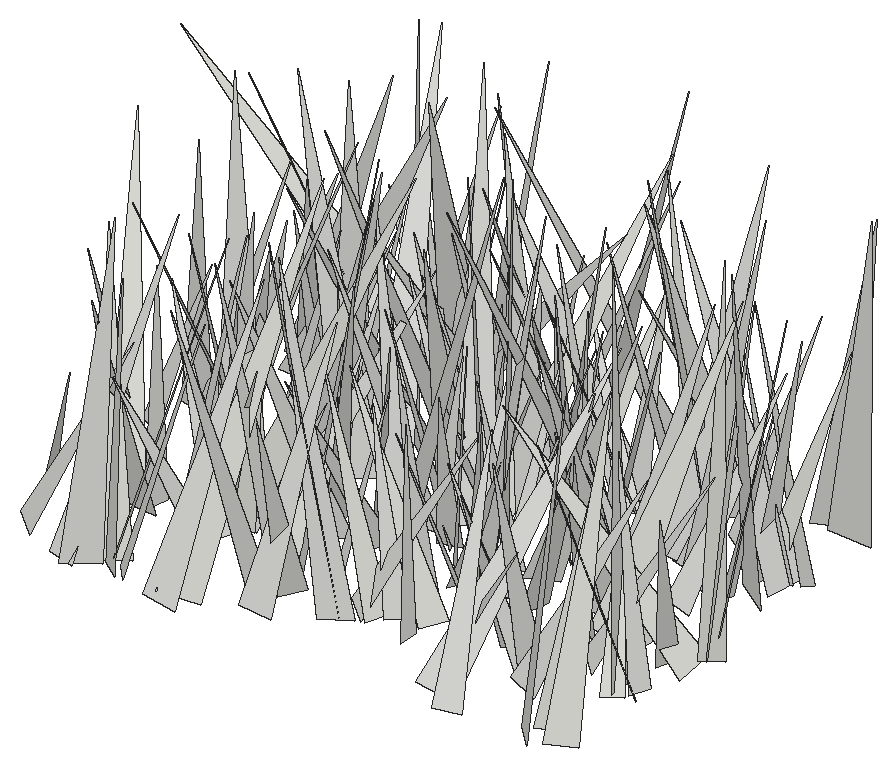
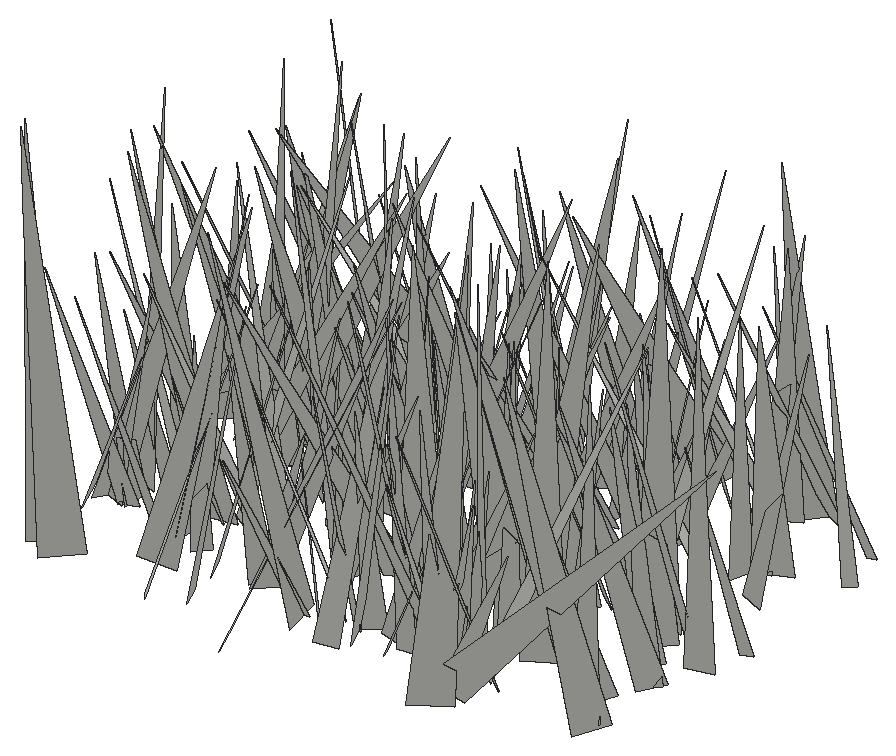
# SketchUp Ruby script. Lengths in inches.
U = 1.inch
M = Sketchup.active_model
def pt(a) = Geom::Point3d.new(a.map { |v| v * U })
def face(e, loops, mat)
  f = e.add_face(loops[0].map { |a| pt(a) })
  loops[1..].each { |l| e.add_face(l.map { |a| pt(a) }).erase! }
  f.material = f.back_material = mat if mat
  f
end
# faces: each face lists its corners as indices into pts; further lists are holes
def faces(e, pts, list, mat = nil) = list.each { |f| face(e, (f[0].is_a?(Array) ? f : [f]).map { |l| l.map { |i| pts[i] } }, mat) }
# xy, xz, yz: faces in a plane at the given z, y or x. An outline is a flat list of corners, or four numbers for a rectangle; further outlines are holes
def ring(l) = l.size == 4 ? [[l[0], l[1]], [l[2], l[1]], [l[2], l[3]], [l[0], l[3]]] : l.each_slice(2).to_a
def flat(e, list, mat, &to3) = list.each { |f| face(e, (f[0].is_a?(Array) ? f : [f]).map { |l| ring(l).map { |u, v| to3.(u, v) } }, mat) }
def xy(e, z, list, mat = nil) = flat(e, list, mat) { |x, y| [x, y, z] }
def xz(e, y, list, mat = nil) = flat(e, list, mat) { |x, z| [x, y, z] }
def yz(e, x, list, mat = nil) = flat(e, list, mat) { |y, z| [x, y, z] }
def lines(e, pts, list) = list.each { |a, b| e.add_line(pt(pts[a]), pt(pts[b])) }
# prism: a flat outline (further loops are holes) pulled along v
def prism(e, loops, v, mat = nil)
  f = face(e, loops, mat); d = Geom::Vector3d.new(v.map { |x| x * U })
  f.pushpull(f.normal.samedirection?(d) ? d.length : -d.length)
end
def box(e, o, s, mat = nil) = prism(e, [[o, [o[0] + s[0], o[1], o[2]], [o[0] + s[0], o[1] + s[1], o[2]], [o[0], o[1] + s[1], o[2]]]], [0, 0, s[2]], mat)
def at(x, y, z, deg = 0) = Geom::Transformation.translation(pt([x, y, z])) * Geom::Transformation.rotation(ORIGIN, Z_AXIS, deg.degrees)
def axes(o, x, y, z) = Geom::Transformation.new([*x, 0, *y, 0, *z, 0, *pt(o).to_a, 1])
def part(name) = M.definitions.add(name)
# library, detail: a bought-in or finely detailed component or shape, given as its bounding box
def library(name, o, s) = part(name).tap { |d| box(d.entities, o, s) }
def detail(e, o, s) = box(e.add_group.entities, o, s)
def put(e, d, t, mat = nil) = e.add_instance(d, t).tap { |i| i.material = mat if mat }
def group(e, t, mat = nil) = e.add_group.tap { |g| g.transformation = t; g.material = mat if mat }.entities
root = M.entities
c1 = part("fur_instance\#9")
p = [[0.8125,0,1.79],[0.67,-0.02,1.48],[0,-0.11,0],[0,0.11,0]]
faces(c1.entities,p,[[0,1,2,3]])
put(root,c1,axes([91.07,234.39,-27.1],[4.75602,-4.66812,2.75377],[-5.20371,-4.95731,0.58378],[-1.51526,2.37234,6.63855]))
put(root,c1,axes([111.02,234.4375,-27.1],[4.54729,4.68314,2.12923],[4.88324,-4.82336,0.17985],[-1.61844,-1.39522,6.52513]))
put(root,c1,axes([92.14,234.72,-27.1],[3.06348,4.37723,2.06786],[4.6001,-3.39453,0.37061],[-1.50841,-1.46222,5.32989]))
put(root,c1,axes([97.12,236.8125,-27.1],[-5.96376,-1.66281,1.60864],[-1.32131,6.09893,1.40577],[1.89916,-0.97833,6.02952]))
put(root,c1,axes([98.24,237.36,-27.1],[3.42227,-3.49613,0.30492],[-3.40506,-3.41104,-0.89344],[-0.84941,-0.41195,4.81005]))
put(root,c1,axes([94.98,233.9,-27.1],[0.10942,6.44965,1.02032],[6.44115,0.06102,-1.07648],[1.07264,-1.02435,6.36012]))
put(root,c1,axes([87.73,235.44,-27.1],[2.82226,4.09729,0.68802],[3.94816,-2.38599,-1.98631],[1.29353,-1.65697,4.56152]))
put(root,c1,axes([107.76,234.14,-27.1],[-1.60174,4.9541,0.61833],[4.97114,1.64265,-0.28364],[0.46172,-0.4996,5.19887]))
put(root,c1,axes([87.05,237.49,-27.1],[4.69242,0.16576,0.10905],[0.19618,-4.2622,-1.96297],[-0.02968,-1.96577,4.26532]))
put(root,c1,axes([92.63,234.77,-27.1],[3.7464,3.46532,0.67043],[3.46985,-3.79505,0.22613],[-0.64655,-0.28736,5.09832]))
put(root,c1,axes([91.81,235.25,-27.1],[-3.36286,5.21282,1.50099],[5.38655,3.41774,0.19865],[0.64152,-1.37145,6.20023]))
put(root,c1,axes([105.42,237.17,-27.1],[3.7363,2.07589,0.22504],[1.88074,-3.14536,-2.2112],[0.90706,-2.02911,3.65784]))
put(root,c1,axes([90.27,238.74,-27.1],[0.60186,-6.09784,0.10298],[-6.0697,-0.58883,0.60707],[0.59415,0.16161,6.09732]))
put(root,c1,axes([93.92,237.96,-27.1],[-4.12735,0.23871,1.0618],[0.66209,3.85593,1.70672],[0.86374,-1.81501,3.76552]))
put(root,c1,axes([98.04,235.48,-27.1],[-0.68675,5.73435,1.62653],[5.78722,1.03346,-1.2],[1.42703,-1.4315,5.64928]))
put(root,c1,axes([108.55,237.99,-27.1],[4.51587,-1.82573,1.61231],[-1.49442,-4.75873,-1.20297],[-1.92343,-0.58918,4.72009]))
put(root,c1,axes([90.3125,234.2,-27.1],[2.22729,6.28936,0.04999],[6.2767,-2.22605,0.40869],[-0.40191,0.08939,6.65956]))
put(root,c1,axes([100.12,237.37,-27.1],[4.02018,4.80904,4.066],[5.52928,-5.00439,0.45193],[-3.01434,-2.76593,6.25176]))
put(root,c1,axes([94.29,235.29,-27.1],[4.06792,5.19434,1.22411],[5.14399,-4.22635,0.83955],[-1.42088,-0.42943,6.54403]))
put(root,c1,axes([100.61,236.82,-27.1],[0.55965,-6.1533,3.26603],[-6.71098,-1.35523,-1.40332],[-1.86889,3.02383,6.01722]))
put(root,c1,axes([112.45,234.71,-27.1],[-5.42402,3.35952,0.54018],[3.08821,5.28712,-1.87283],[1.42868,1.32596,6.09909]))
put(root,c1,axes([106.79,239.1,-27.1],[1.2889,-4.23263,0.01136],[-4.22076,-1.28617,-0.32791],[-0.31699,-0.08469,4.41236]))
put(root,c1,axes([111.32,235.29,-27.1],[-4.3486,2.21974,0.80785],[1.83051,4.23636,-1.78683],[1.49303,1.27131,4.54366]))
put(root,c1,axes([103.45,237.36,-27.1],[-3.94466,-0.14605,1.57067],[-0.23954,4.23653,-0.20765],[1.55915,0.28136,3.94189]))
put(root,c1,axes([111.99,239.29,-27.1],[-3.65311,-4.50937,0.62916],[-4.48426,3.70309,0.50402],[0.78847,0.16789,5.78149]))
put(root,c1,axes([108.77,237.1,-27.1],[0.87918,5.14411,1.43079],[4.85097,-0.16366,-2.39235],[2.23095,-1.67133,4.63805]))
put(root,c1,axes([108.61,237.67,-27.1],[-0.27177,-3.75184,1.87256],[-3.70908,-0.66019,-1.86105],[-1.95589,1.77327,3.26904]))
put(root,c1,axes([96.52,238.8,-27.1],[-6.02473,-0.71032,1.74625],[-0.51818,6.24626,0.75302],[1.81257,-0.57532,6.01954]))
put(root,c1,axes([101.71,237.83,-27.1],[-4.44101,1.77663,0.66677],[1.83519,4.45274,0.3588],[0.48276,-0.58331,4.76973]))
put(root,c1,axes([106.6,234.94,-27.1],[-2.65177,6.66161,0.65253],[5.97681,2.67255,-2.995],[3.01341,0.56142,6.51452]))
put(root,c1,axes([100.72,237.83,-27.1],[2.95433,4.07724,0.35212],[3.82019,-2.59183,-2.04072],[1.46767,-1.46099,4.60298]))
put(root,c1,axes([93.55,238.49,-27.1],[4.21997,-0.6182,0.41958],[-0.60999,-4.24047,-0.11271],[-0.43142,-0.05127,4.26352]))
put(root,c1,axes([104.69,239.23,-27.1],[5.27182,0.13194,1.25121],[0.40362,-5.28245,-1.14356],[-1.19165,-1.2055,5.14798]))
put(root,c1,axes([95.3,234.58,-27.1],[-5.76444,5.45156,1.05869],[4.71185,5.60881,-3.22628],[2.93919,1.70025,7.24841]))
put(root,c1,axes([102.25,238.19,-27.1],[-2.34318,3.21724,1.23905],[3.43189,2.31946,0.46753],[0.3286,-1.2829,3.95253]))
put(root,c1,axes([91.68,235.6,-27.1],[4.88269,3.53574,0.69101],[3.04894,-4.67553,2.3797],[-1.91908,1.56767,5.53887]))
put(root,c1,axes([103.54,238.68,-27.1],[-3.16425,3.77948,0.90882],[3.82647,2.82214,1.58634],[-0.68447,-1.69527,4.66695]))
put(root,c1,axes([90.54,239.28,-27.1],[4.66089,-0.94094,1.87831],[-0.93791,-5.02216,-0.1885],[-1.87983,0.17273,4.75118]))
put(root,c1,axes([99.8,237.57,-27.1],[2.15657,3.40289,0.33157],[3.29952,-2.17412,0.8525],[-0.89598,0.18416,3.93747]))
put(root,c1,axes([93.79,238.93,-27.1],[-4.37438,2.14658,0.79892],[2.22863,4.38643,0.41683],[0.52851,-0.72986,4.85482]))
put(root,c1,axes([106.63,236.22,-27.1],[4.76717,4.34009,0.09976],[4.0907,-4.54047,2.05487],[-1.45344,1.45601,6.11063]))
put(root,c1,axes([104.82,239.42,-27.1],[-3.19994,-2.12817,0.10035],[-2.08753,3.09569,-0.91527],[-0.42587,0.81635,3.73243]))
put(root,c1,axes([94.13,239.69,-27.1],[2.50338,-2.82714,1.30611],[-3.05988,-2.54469,0.35667],[-0.57944,1.22368,3.75931]))
put(root,c1,axes([89.07,240.52,-27.1],[-1.67954,-4.60165,1.09216],[-4.72861,1.65608,-0.29411],[0.09072,1.12742,4.88974]))
put(root,c1,axes([93.97,240.62,-27.1],[-1.02707,-3.52995,0.46815],[-3.49734,0.90838,-0.82343],[-0.66956,0.66999,3.58293]))
put(root,c1,axes([101.92,240.24,-27.1],[0.28904,-4.61969,1.68996],[-4.89331,-0.44312,-0.3744],[-0.50298,1.65624,4.61355]))
put(root,c1,axes([111.68,238.54,-27.1],[-2.57238,2.98987,0.10946],[2.97729,2.57237,-0.29516],[0.29502,0.10983,3.93311]))
put(root,c1,axes([98.65,241.95,-27.1],[1.56687,-4.2825,0.24372],[-4.04586,-1.5617,-1.43053],[-1.42486,-0.27491,4.32996]))
put(root,c1,axes([112.21,239.42,-27.1],[-4.36363,0.98227,0.81119],[0.91976,4.432,-0.41906],[0.88144,0.23814,4.45315]))
put(root,c1,axes([97.375,238.89,-27.1],[5.30824,4.83924,1.79848],[4.88732,-5.54151,0.48577],[-1.6634,-0.83881,7.16657]))
put(root,c1,axes([97.09,241.42,-27.1],[0.61294,-5.47928,1.38132],[-5.30961,-1.0339,-1.7451],[-1.93355,1.10218,5.22999]))
put(root,c1,axes([111.69,241.67,-27.1],[3.7269,-2.05729,0.24824],[-1.97365,-3.67974,-0.86491],[-0.63149,-0.64103,4.16823]))
put(root,c1,axes([112.61,241.98,-27.1],[-5.96221,1.49508,0.02596],[1.36332,5.39133,2.61894],[-0.61423,-2.54602,5.56097]))
put(root,c1,axes([109.48,239.97,-27.1],[3.29682,4.04593,0.27696],[3.82738,-2.98619,-1.93627],[1.34069,-1.42422,4.84659]))
put(root,c1,axes([111.5,239.28,-27.1],[-7.33304,-1.55705,2.53328],[-2.07568,7.50758,-1.39398],[2.1292,1.95633,7.36578]))
put(root,c1,axes([107.93,241.74,-27.1],[-3.27673,-6.38483,2.25273],[-6.55108,3.62196,0.73666],[1.71005,1.64109,7.13865]))
put(root,c1,axes([96.43,242.04,-27.1],[6.1777,-0.38175,1.16241],[-0.13775,-6.16226,-1.29169],[-1.21571,-1.24165,6.0532]))
put(root,c1,axes([108.61,243.0625,-27.1],[1.25653,-6.81976,0.6894],[-6.81087,-1.32116,-0.65555],[-0.77223,0.55558,6.90349]))
put(root,c1,axes([89.71,238.5,-27.1],[-3.35316,6.39569,0.22234],[6.39729,3.34326,0.30873],[-0.17041,-0.34016,7.2148]))
put(root,c1,axes([92.72,241.87,-27.1],[-4.52954,-3.25843,1.35312],[-3.24257,4.71245,0.49358],[1.39071,0.3748,5.55792]))
put(root,c1,axes([90.9,244.39,-27.1],[-3.5223,-6.70382,0.02091],[-6.50166,3.42181,1.83516],[1.63401,-0.83562,7.34711]))
put(root,c1,axes([105.59,241.77,-27.1],[5.75538,-1.33671,0.29214],[-1.31847,-5.75568,-0.36093],[-0.36579,-0.28603,5.89753]))
put(root,c1,axes([96.39,239.39,-27.1],[-0.08905,4.06249,0.07241],[4.03019,0.09752,-0.5148],[0.51634,-0.06053,4.03072]))
put(root,c1,axes([96.22,240.78,-27.1],[6.38411,4.40631,2.11358],[4.61615,-6.57865,-0.22824],[-1.60436,-1.39477,7.75373]))
put(root,c1,axes([97.61,242.99,-27.1],[4.97524,0.71585,1.07536],[1.04452,-4.74693,-1.67259],[-0.76015,-1.83742,4.74004]))
put(root,c1,axes([110.31,242.54,-27.1],[-3.89042,0.9571,1.21715],[1.27935,3.84105,1.06884],[0.87221,-1.36496,3.86121]))
put(root,c1,axes([93.42,240.59,-27.1],[2.59444,7.48207,1.23534],[7.31718,-2.12705,-2.48457],[1.99156,-1.93206,7.51927]))
put(root,c1,axes([100.42,243.47,-27.1],[1.67975,-3.93598,0.16611],[-3.93538,-1.66827,0.26597],[0.17974,0.25696,4.27115]))
put(root,c1,axes([100.32,241.13,-27.1],[-1.21025,6.4146,1.42422],[6.45546,0.89059,1.47445],[-1.22575,-1.64315,6.35907]))
put(root,c1,axes([91.96,239.77,-27.1],[5.80303,5.01805,0.27093],[4.96083,-5.78629,0.91567],[-0.80277,0.51711,7.61693]))
put(root,c1,axes([107.73,242.9,-27.1],[0.85171,-3.4207,0.8533],[-3.50883,-0.73716,0.54719],[0.34265,0.95401,3.48241]))
put(root,c1,axes([101.58,242.3125,-27.1],[3.14318,2.78213,1.66083],[2.96777,-3.40061,0.07991],[-1.30037,-1.03624,4.19683]))
put(root,c1,axes([103.09,241.92,-27.1],[4.37398,5.97616,2.1686],[6.29129,-4.44766,-0.43255],[-0.91492,-2.01317,7.39318]))
put(root,c1,axes([102.34,241.34,-27.1],[4.56042,0.58445,0.815],[0.35248,-4.48653,1.24501],[-0.93891,1.15443,4.42595]))
put(root,c1,axes([100.34,243.73,-27.1],[-4.23671,-2.59002,0.97553],[-2.55905,4.34534,0.42292],[1.0541,0.13924,4.94763]))
put(root,c1,axes([104.03,242.01,-27.1],[-6.60957,-3.13791,3.29203],[-3.79035,7.01015,-0.92809],[2.51341,2.31982,7.25752]))
put(root,c1,axes([98.69,244.4,-27.1],[-5.81258,-1.56867,1.18702],[-1.32265,5.85738,1.26392],[1.45614,-0.94136,5.88637]))
put(root,c1,axes([100.27,240.39,-27.1],[7.12046,1.58475,2.39098],[0.70942,-7.17277,2.64146],[-2.77938,2.22916,6.79964]))
put(root,c1,axes([103.33,243.52,-27.1],[-0.82021,3.34867,1.94688],[3.86928,0.61559,0.57127],[-0.18046,-2.02092,3.4]))
put(root,c1,axes([108.05,244.6,-27.1],[-2.49506,-7.82927,1.12782],[-7.54738,2.00233,-2.79687],[-2.3678,1.86761,7.7266]))
put(root,c1,axes([94.34,241.92,-27.1],[1.81357,5.35205,0.20733],[5.12174,-1.66889,-1.72019],[1.56691,-0.73948,5.38279]))
put(root,c1,axes([93.54,244.82,-27.1],[5.39011,-5.98506,0.75501],[-6.02641,-5.29691,1.03406],[0.27067,1.25142,7.9878]))
put(root,c1,axes([108.91,241.81,-27.1],[-0.63507,6.95916,1.46669],[6.78735,1.03289,-1.962],[2.12438,-1.21968,6.70699]))
put(root,c1,axes([104.47,243.61,-27.1],[5.13759,-3.83835,0.8309],[-3.9202,-4.93031,1.46363],[0.23526,1.66651,6.24384]))
put(root,c1,axes([104.13,241.83,-27.1],[0.66695,4.37993,0.08385],[4.36286,-0.67176,0.3871],[-0.39533,-0.02429,4.41347]))
put(root,c1,axes([95.62,243.7,-27.1],[-2.49049,-3.07283,1.62396],[-3.33154,2.67981,-0.03854],[0.99012,1.28779,3.95516]))
put(root,c1,axes([89.54,244.43,-27.1],[3.73813,0.01426,0.67221],[0.17612,-3.68545,-0.90117],[-0.64889,-0.91811,3.62791]))
put(root,c1,axes([86.79,243.62,-27.1],[-0.2038,-3.57727,1.86557],[-3.68837,0.92217,1.36537],[1.63497,1.63446,3.31273]))
put(root,c1,axes([99.51,243.89,-27.1],[1.31397,-3.56018,1.31098],[-3.78942,-1.16427,0.63629],[0.18405,1.44556,3.7412]))
put(root,c1,axes([108.75,244.44,-27.1],[-4.44374,-5.75342,0.61079],[-5.6055,4.0905,-2.25122],[-1.43294,1.84058,6.91236]))
put(root,c1,axes([94.58,244.43,-27.1],[3.50873,2.55931,1.93983],[3.03472,-3.58228,-0.76287],[-1.05048,-1.80039,4.27543]))
put(root,c1,axes([89.55,244.97,-27.1],[3.84963,-3.94903,0.87916],[-4.01863,-3.87266,0.20133],[-0.4673,0.77142,5.51126]))
put(root,c1,axes([90.29,244.34,-27.1],[4.03772,-5.94106,3.0996],[-6.44975,-4.42725,-0.08397],[-1.8178,2.512,7.18278]))
put(root,c1,axes([98.27,246.61,-27.1],[2.21636,-6.61774,0.25451],[-6.61771,-2.20273,0.35418],[0.25535,0.35358,6.97003]))
put(root,c1,axes([104.12,245.55,-27.1],[-2.04339,-2.88899,0.9747],[-2.5158,2.26047,1.42575],[1.7225,-0.12566,3.23866]))
put(root,c1,axes([102.68,242.01,-27.1],[-0.48607,6.36101,0.33267],[6.36907,0.48063,0.1158],[-0.09028,-0.34048,6.37851]))
put(root,c1,axes([87.42,245.51,-27.1],[0.11264,-6.37998,1.60761],[-6.5012,0.13924,1.0081],[1.01142,1.60553,6.30084]))
put(root,c1,axes([99.97,245.76,-27.1],[-2.55131,-7.67351,1.38924],[-7.65133,2.18082,-2.00574],[-1.50657,1.91917,7.83383]))
put(root,c1,axes([92.95,243.73,-27.1],[3.70587,4.25797,0.60198],[4.28884,-3.60158,-0.92773],[0.31394,-1.06043,5.56805]))
put(root,c1,axes([105.88,243.91,-27.1],[2.53366,4.26731,1.78001],[4.34271,-2.89305,0.75426],[-1.5872,-1.10369,4.90515]))
put(root,c1,axes([92.89,242.58,-27.1],[-4.41851,1.16155,1.66424],[0.34777,4.36157,-2.12081],[1.99949,1.8082,4.04655]))
put(root,c1,axes([106.66,247.26,-27.1],[-4.09518,-5.32392,0.52178],[-5.17841,4.11019,1.29512],[1.34181,-0.38619,6.5907]))
put(root,c1,axes([94.41,243.63,-27.1],[1.13394,4.06883,0.24777],[4.07369,-1.14042,0.08414],[-0.14769,-0.216,4.22305]))
put(root,c1,axes([88.21,244.77,-27.1],[3.54049,4.95211,1.34575],[5.12044,-3.30078,-1.32493],[0.33991,-1.85767,5.94164]))
put(root,c1,axes([104.58,247.31,-27.1],[6.71484,1.18998,0.43364],[1.2609,-6.06064,-2.89345],[0.11927,-2.92333,6.1752]))
put(root,c1,axes([101.95,243.55,-27.1],[-6.04222,-2.58238,2.07365],[-3.21518,5.60869,-2.38377],[0.79453,3.05796,6.1233]))
put(root,c1,axes([94.92,245.3125,-27.1],[1.79805,-6.87497,3.712],[-7.43664,-2.674,-1.35027],[-2.39594,3.14033,6.97674]))
put(root,c1,axes([112.47,242.65,-27.1],[3.51213,5.3509,1.08193],[4.75447,-3.63032,2.52063],[-2.68285,0.57134,5.88334]))
put(root,c1,axes([107.41,244.48,-27.1],[1.23681,5.98503,1.54047],[6.1022,-0.934,-1.27052],[0.97821,-1.7408,5.97797]))
put(root,c1,axes([112.8,242.75,-27.1],[-7.06937,0.92542,0.80535],[0.55425,6.6114,-2.73188],[1.09444,2.62944,6.58553]))
put(root,c1,axes([88.97,246.28,-27.1],[3.21186,-3.52218,0.8528],[-3.62385,-3.13,0.72104],[-0.02677,1.11644,4.71189]))
put(root,c1,axes([88.02,247.55,-27.1],[0.93957,-4.99379,0.05949],[-4.70596,-0.86502,1.71172],[1.67197,0.37157,4.78443]))
put(root,c1,axes([96.04,248.03,-27.1],[-1.10699,-6.38687,0.31821],[-6.26084,1.01671,-1.37367],[-1.30201,0.54128,6.33487]))
put(root,c1,axes([111.6875,244.67,-27.1],[-4.45958,-2.36263,3.46386],[-3.3219,5.07642,-0.81428],[2.55838,2.47306,4.98064]))
put(root,c1,axes([111.05,247.21,-27.1],[-3.13728,-6.42445,2.27927],[-6.51063,3.56742,1.09378],[2.01998,1.52023,7.06539]))
put(root,c1,axes([99.96,245.46,-27.1],[-1.66543,4.2087,0.7623],[4.0491,1.28782,1.73616],[-1.37806,-1.30242,4.18002]))
put(root,c1,axes([94.3,247.96,-27.1],[-0.53016,-5.209,0.61736],[-4.97847,0.69512,1.58982],[1.65216,0.4231,4.98871]))
put(root,c1,axes([109.42,245.03,-27.1],[0.30593,5.01742,0.69432],[4.86404,-0.09691,-1.44288],[1.4134,-0.75252,4.8152]))
put(root,c1,axes([91.51,247.65,-27.1],[4.6906,-0.13116,1.94102],[0.35682,-4.92253,-1.19491],[-1.91244,-1.24013,4.53774]))
put(root,c1,axes([93.81,248.23,-27.1],[5.31663,-1.02418,0.76649],[-0.77202,-5.18142,-1.56841],[-1.02002,-1.41668,5.18224]))
put(root,c1,axes([102.05,247.5,-27.1],[6.71325,2.37054,1.67819],[2.73448,-6.58312,-1.63968],[-0.97898,-2.13225,6.9281]))
put(root,c1,axes([97.625,247.47,-27.1],[3.16597,-2.82128,1.36449],[-2.73379,-3.43456,-0.75836],[-1.53229,0.2984,4.17228]))
put(root,c1,axes([98.09,248.09,-27.1],[2.45481,-4.16097,0.8917],[-4.06011,-2.59844,-0.9479],[-1.27449,0.26329,4.73722]))
put(root,c1,axes([110.41,246.6,-27.1],[3.57631,0.31891,0.97988],[0.16002,-3.66803,0.60973],[-1.01797,0.54376,3.53835]))
put(root,c1,axes([97.04,248.83,-27.1],[-3.71631,2.59474,2.95715],[3.6126,3.86147,1.15179],[1.55775,-2.76492,4.38373]))
put(root,c1,axes([100.15,245.23,-27.1],[-7.18499,4.19207,1.05141],[4.04317,7.24035,-1.23823],[1.52698,0.55406,8.22584]))
put(root,c1,axes([101,247.6,-27.1],[-6.55699,2.55506,2.62376],[2.8465,6.94107,0.35432],[2.30431,-1.30376,7.02829]))
put(root,c1,axes([108.68,246.88,-27.1],[3.30058,6.51639,2.13105],[6.85171,-3.21879,-0.76942],[-0.24255,-2.25268,7.26396]))
put(root,c1,axes([92.1,248.44,-27.1],[3.60415,-6.43604,2.10161],[-6.7075,-3.71823,0.11619],[-0.92131,1.89247,7.37557]))
put(root,c1,axes([104.625,246.95,-27.1],[-5.51822,-0.21879,0.79161],[-0.32668,5.51842,-0.75206],[0.75352,0.79022,5.4711]))
put(root,c1,axes([87.93,247.53,-27.1],[2.95683,-4.48742,1.40063],[-4.613,-2.45121,1.88504],[0.90496,2.16707,5.03253]))
put(root,c1,axes([96.84,251.42,-27.1],[-5.64756,-4.03637,0.24701],[-3.60758,5.22048,2.82493],[1.82721,-2.16853,6.3409]))
put(root,c1,axes([111.53,248.54,-27.1],[-7.04891,1.70289,1.4017],[1.92518,7.04086,1.12767],[1.07622,-1.44158,7.16347]))
put(root,c1,axes([102.21,247.46,-27.1],[-3.53666,-0.44387,1.07965],[-0.6619,3.59984,-0.68824],[0.96154,0.84544,3.49732]))
put(root,c1,axes([92.99,246.96,-27.1],[2.64907,4.14771,0.84835],[4.17625,-2.72433,0.27885],[-0.69438,-0.56151,4.91358]))
put(root,c1,axes([101.12,248.55,-27.1],[-2.05485,-3.90462,0.97999],[-3.96047,1.76344,-1.27819],[-0.72186,1.43981,4.22312]))
put(root,c1,axes([96.21,248.88,-27.1],[-2.14589,-4.13922,0.79032],[-4.13009,1.88974,-1.31675],[-0.83673,1.28775,4.4726]))
put(root,c1,axes([98.83,252.27,-27.1],[-2.64275,-7.72517,0.10148],[-7.35563,2.5487,2.46402],[2.36287,-0.70608,7.78402]))
put(root,c1,axes([93.26,250.15,-27.1],[-4.92734,-5.46841,0.2776],[-5.45988,4.87887,-0.80338],[-0.41255,0.74316,7.31688]))
put(root,c1,axes([111.28,248.71,-27.1],[-0.94166,-4.10224,1.61468],[-4.38512,0.70145,-0.77524],[-0.45421,1.73259,4.13692]))
put(root,c1,axes([108.26,248.75,-27.1],[-6.28358,-3.49392,1.76213],[-3.72095,6.36668,-0.64478],[1.21124,1.43309,7.16066]))
put(root,c1,axes([110.57,248.31,-27.1],[4.80103,-0.44543,1.50068],[-0.59366,-4.99749,0.41591],[-1.44845,0.57184,4.80368]))
put(root,c1,axes([88.14,251.01,-27.1],[0.06322,-6.05576,0.15688],[-5.74231,-0.00994,1.93043],[1.92942,0.16885,5.74018]))
put(root,c1,axes([106.89,246.5,-27.1],[5.00084,3.55671,0.83126],[3.26277,-4.98345,1.69387],[-1.6418,0.92989,5.89825]))
put(root,c1,axes([95.6,245.87,-27.1],[-4.43994,6.98412,0.3729],[6.94517,4.45476,-0.74146],[0.82561,0.08476,8.24265]))
put(root,c1,axes([106.48,249.69,-27.1],[3.38817,-1.89067,0.4047],[-1.85762,-3.4096,-0.37677],[-0.53632,-0.13453,3.86165]))
put(root,c1,axes([107.46,247.53,-27.1],[1.47589,3.3854,0.35503],[3.34161,-1.51469,0.55196],[-0.64858,-0.1002,3.65165]))
put(root,c1,axes([107.42,247.6,-27.1],[0.16612,7.76506,1.97129],[7.95416,0.07536,-0.96713],[0.95574,-1.97685,7.70638]))
put(root,c1,axes([99.72,250.33,-27.1],[-3.13954,-2.86345,1.03549],[-2.74612,3.30524,0.81394],[1.31545,0.06589,4.17056]))
put(root,c1,axes([88.87,249.58,-27.1],[4.47531,-6.51665,1.20055],[-6.35255,-3.80729,3.0143],[1.88498,2.64087,7.30815]))
put(root,c1,axes([103.07,250.37,-27.1],[-6.35837,1.48,1.02188],[1.69793,6.17763,1.61781],[0.593,-1.81932,6.3247]))
put(root,c1,axes([96.82,249.21,-27.1],[3.38987,-1.12165,1.00676],[-1.27426,-3.45624,0.43994],[-0.80492,0.7478,3.54341]))
put(root,c1,axes([110.53,248.75,-27.1],[0.61438,4.77457,1.24038],[4.786,-0.27399,-1.3159],[1.1955,-1.35681,4.63059]))
put(root,c1,axes([99.86,246.79,-27.1],[0.36828,7.38641,0.21711],[7.15433,-0.30198,-1.86176],[1.84979,-0.30261,7.15741]))
put(root,c1,axes([96.3125,250.84,-27.1],[-1.36067,-5.7583,1.83351],[-5.61411,1.9,1.80082],[2.23642,1.26617,5.63617]))
put(root,c1,axes([103.92,249.1875,-27.1],[-2.71204,2.5664,0.21286],[2.56651,2.66825,0.52947],[-0.21147,-0.53003,3.69611]))
put(root,c1,axes([107.15,251.4,-27.1],[1.49882,-6.76146,1.59023],[-6.75855,-1.79498,-1.262],[-1.60255,1.24632,6.80963]))
put(root,c1,axes([100.41,250.72,-27.1],[3.23905,1.92957,1.10614],[2.22288,-2.8741,-1.49551],[-0.07469,-1.85863,3.46094]))
put(root,c1,axes([98.2,250.3,-27.1],[2.26375,-3.28304,0.92587],[-3.40814,-2.22313,0.4499],[-0.14199,1.01955,3.96238]))
put(root,c1,axes([97.3125,250.49,-27.1],[-0.77658,-4.10323,1.17838],[-4.23531,0.59015,-0.73621],[-0.53592,1.28194,4.11067]))
put(root,c1,axes([105.3,250.46,-27.1],[-4.90258,-2.23132,0.87524],[-2.28191,4.95484,-0.15015],[0.73329,0.50088,5.38438]))
put(root,c1,axes([107.61,248.76,-27.1],[-6.80477,1.06742,0.77743],[0.9228,6.76292,-1.20833],[0.94457,1.0827,6.78117]))
put(root,c1,axes([94.0625,251.35,-27.1],[5.26826,5.58359,0.80335],[4.69893,-3.73546,-4.8521],[3.1212,-3.80083,5.9488]))
put(root,c1,axes([93.42,250.21,-27.1],[4.5767,5.68819,3.18986],[6.17982,-5.02762,0.09872],[-2.08339,-2.41752,7.30013]))
put(root,c1,axes([103.42,250.07,-27.1],[3.51253,-2.51047,1.78394],[-2.89575,-3.6135,0.61652],[-1.0486,1.56939,4.2732]))
put(root,c1,axes([93.25,253.37,-27.1],[6.31463,-5.10403,0.36931],[-4.97216,-6.25818,-1.47472],[-1.21044,-0.91981,7.98441]))
put(root,c1,axes([93.05,251.71,-27.1],[3.48904,-1.79502,0.75996],[-1.60226,-3.52839,-0.97792],[-1.11014,-0.54905,3.7999]))
put(root,c1,axes([112.08,249.07,-27.1],[-5.07583,-0.99149,0.0646],[-0.93064,4.62637,-2.11704],[-0.34804,2.08923,4.7186]))
put(root,c1,axes([98.78,250.5625,-27.1],[2.69077,3.3772,1.27263],[3.60609,-2.57991,-0.77814],[-0.14558,-1.48455,4.24737]))
put(root,c1,axes([108.22,249.82,-27.1],[2.30047,4.4169,0.81433],[4.47004,-2.16262,-0.89782],[0.43686,-1.13065,4.89848]))
put(root,c1,axes([106,253.49,-27.1],[-4.51609,-3.87484,0.43498],[-3.47065,4.29803,2.25393],[1.77713,-1.453,5.5072]))
put(root,c1,axes([97.33,249,-27.1],[4.31579,6.0344,1.65644],[5.97789,-4.5707,1.07586],[-1.85004,-0.69181,7.34048]))
put(root,c1,axes([93.36,251.74,-27.1],[0.28978,-3.77503,0.68612],[-3.83038,-0.24462,0.27184],[0.22308,0.70349,3.77636]))
put(root,c1,axes([98.49,250.96,-27.1],[5.38161,2.47127,3.67462],[2.66712,-6.4254,0.41515],[-3.53503,-1.08568,5.90733]))
put(root,c1,axes([87.71,251.2,-27.1],[5.60342,-3.67276,1.04707],[-3.81273,-5.48708,1.15708],[-0.22057,1.54484,6.59914]))
put(root,c1,axes([99.76,250.08,-27.1],[4.90909,4.36789,0.50992],[4.39704,-4.86378,-0.66882],[0.06695,-0.83837,6.53684]))
put(root,c1,axes([95.2,250.04,-27.1],[-4.58169,-0.00231,0.33908],[-0.10273,4.38765,-1.35823],[0.32316,1.36211,4.37574]))
put(root,c1,axes([93.56,252.18,-27.1],[-5.86481,5.71927,0.12396],[4.62698,4.63811,4.91939],[-3.36399,-3.59156,6.55024]))
put(root,c1,axes([111.08,252.64,-27.1],[1.84601,-7.44066,1.73932],[-7.59322,-1.58595,1.27441],[0.85535,1.97933,7.55956]))
put(root,c1,axes([104.71,252.54,-27.1],[4.53456,1.85789,3.16607],[2.55783,-5.20835,-0.60709],[-2.63311,-1.85992,4.86266]))
put(root,c1,axes([93.76,252.22,-27.1],[0.23103,-4.99246,1.62863],[-5.17408,0.0623,0.92493],[0.89778,1.64376,4.91147]))
put(root,c1,axes([110.09,253.04,-27.1],[4.60789,-6.31495,1.14074],[-6.41656,-4.51508,0.92427],[0.08686,1.46561,7.76253]))
put(root,c1,axes([100.75,251.23,-27.1],[7.58691,1.58366,1.76713],[1.48707,-7.78642,0.59349],[-1.84915,0.23586,7.72768]))
put(root,c1,axes([93.61,251.7,-27.1],[-2.38468,3.13652,0.12042],[3.02513,2.25628,1.13874],[-0.83714,-0.7813,3.77197]))
put(root,c1,axes([101.76,254.36,-27.1],[-6.74137,-3.47517,0.05647],[-3.44773,6.70195,0.85032],[0.43951,-0.73012,7.53656]))
put(root,c1,axes([92.57,250.65,-27.1],[3.35621,4.76804,0.53975],[4.75729,-3.3924,0.38655],[-0.62744,-0.21695,5.81798]))
put(root,c1,axes([100.91,251.06,-27.1],[0.42201,3.83383,0.13948],[3.79822,-0.3978,-0.55775],[0.53966,-0.19825,3.81644]))
put(root,c1,axes([94.56,250.9,-27.1],[3.67967,2.76321,1.03507],[2.46473,-3.78797,1.35021],[-1.62229,0.51247,4.39911]))
